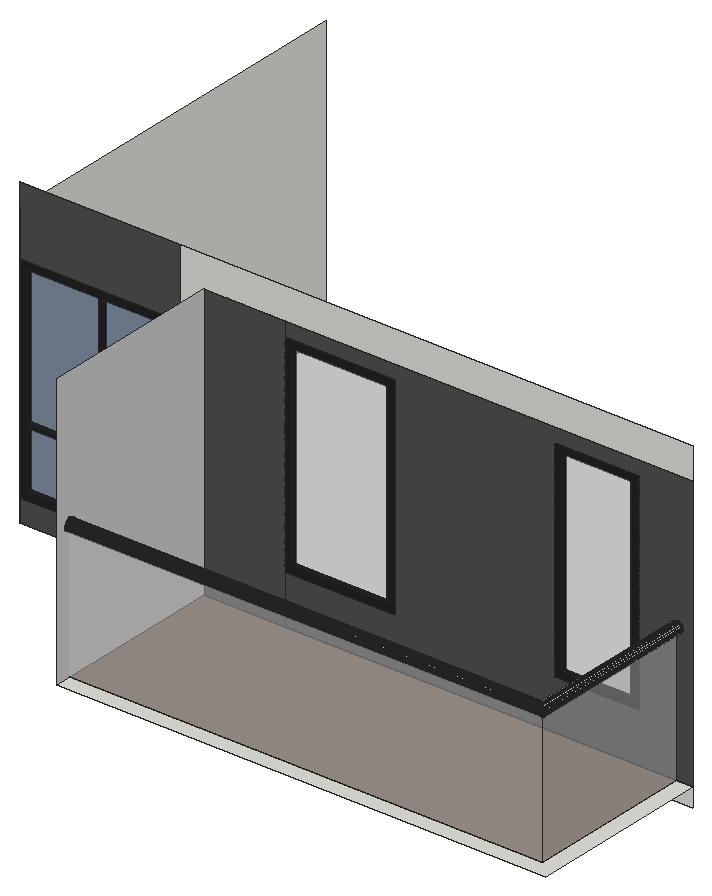
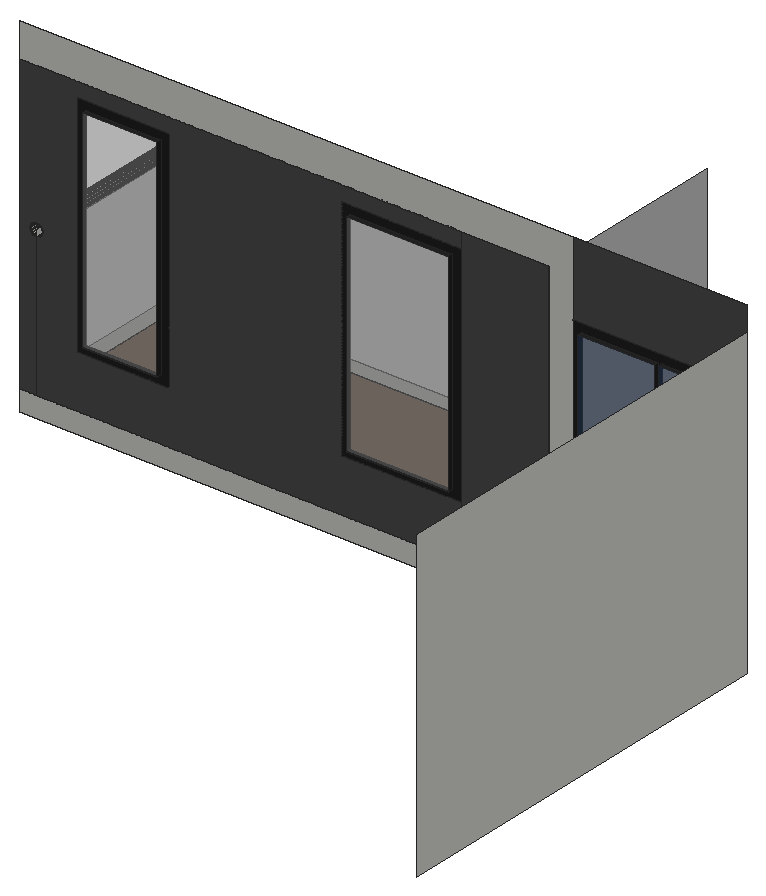
# SketchUp Ruby script. Lengths in inches.
U = 1.inch
M = Sketchup.active_model
def pt(a) = Geom::Point3d.new(a.map { |v| v * U })
def face(e, loops, mat)
  f = e.add_face(loops[0].map { |a| pt(a) })
  loops[1..].each { |l| e.add_face(l.map { |a| pt(a) }).erase! }
  f.material = f.back_material = mat if mat
  f
end
# faces: each face lists its corners as indices into pts; further lists are holes
def faces(e, pts, list, mat = nil) = list.each { |f| face(e, (f[0].is_a?(Array) ? f : [f]).map { |l| l.map { |i| pts[i] } }, mat) }
# xy, xz, yz: faces in a plane at the given z, y or x. An outline is a flat list of corners, or four numbers for a rectangle; further outlines are holes
def ring(l) = l.size == 4 ? [[l[0], l[1]], [l[2], l[1]], [l[2], l[3]], [l[0], l[3]]] : l.each_slice(2).to_a
def flat(e, list, mat, &to3) = list.each { |f| face(e, (f[0].is_a?(Array) ? f : [f]).map { |l| ring(l).map { |u, v| to3.(u, v) } }, mat) }
def xy(e, z, list, mat = nil) = flat(e, list, mat) { |x, y| [x, y, z] }
def xz(e, y, list, mat = nil) = flat(e, list, mat) { |x, z| [x, y, z] }
def yz(e, x, list, mat = nil) = flat(e, list, mat) { |y, z| [x, y, z] }
def lines(e, pts, list) = list.each { |a, b| e.add_line(pt(pts[a]), pt(pts[b])) }
# prism: a flat outline (further loops are holes) pulled along v
def prism(e, loops, v, mat = nil)
  f = face(e, loops, mat); d = Geom::Vector3d.new(v.map { |x| x * U })
  f.pushpull(f.normal.samedirection?(d) ? d.length : -d.length)
end
def box(e, o, s, mat = nil) = prism(e, [[o, [o[0] + s[0], o[1], o[2]], [o[0] + s[0], o[1] + s[1], o[2]], [o[0], o[1] + s[1], o[2]]]], [0, 0, s[2]], mat)
def at(x, y, z, deg = 0) = Geom::Transformation.translation(pt([x, y, z])) * Geom::Transformation.rotation(ORIGIN, Z_AXIS, deg.degrees)
def axes(o, x, y, z) = Geom::Transformation.new([*x, 0, *y, 0, *z, 0, *pt(o).to_a, 1])
def part(name) = M.definitions.add(name)
# library, detail: a bought-in or finely detailed component or shape, given as its bounding box
def library(name, o, s) = part(name).tap { |d| box(d.entities, o, s) }
def detail(e, o, s) = box(e.add_group.entities, o, s)
def put(e, d, t, mat = nil) = e.add_instance(d, t).tap { |i| i.material = mat if mat }
def group(e, t, mat = nil) = e.add_group.tap { |g| g.transformation = t; g.material = mat if mat }.entities
root = M.entities
M.materials.add("[0136_Charcoal]").color = [35, 35, 35]
M.materials.add("[Cladding Siding White]2").color = [81, 81, 81]
M.materials.add("[Cladding Siding White]3").color = [207, 207, 207]
M.materials.add("[Granite Brown]").color = [126, 104, 91]
M.materials.add("[Translucent Glass Blue]").color = [52, 78, 124]
M.materials["[Translucent Glass Blue]"].alpha = 0.5
M.materials.add("[Translucent Glass Gray]").color = [211, 211, 211]
M.materials["[Translucent Glass Gray]"].alpha = 0.5
M.materials.add("[Translucent Glass Gray]1").color = [163, 163, 163]
M.materials["[Translucent Glass Gray]1"].alpha = 0.5
xy(root,883.9375,[[559.63,120.38,558.375,120.39,557.125,120.53,555.9,120.8,554.71,121.2,553.5625,121.72,552.48,122.35,551.47,123.1,550.54,123.95,549.71,124.89,548.98,125.91,548.36,127,547.86,128.15,547.48,129.35,547.23,130.58,547.1,131.83,547.11,133.09,547.25,134.33,547.52,135.56,547.92,136.75,548.44,137.9,549.08,138.98,549.82,139.99,550.67,140.92,551.61,141.75,552.63,142.48,553.72,143.1,554.875,143.6,556.07,143.98,557.3,144.23,558.55,144.35,559.81,144.35,561.06,144.2,562.28,143.93,563.48,143.54,564.62,143.02,565.7,142.38,566.71,141.64,567.64,140.79,568.47,139.85,569.2,138.83,569.82,137.73,570.33,136.58,570.71,135.39,570.96,134.15,571.08,132.9,571.07,131.65,570.93,130.4,570.66,129.17,570.26,127.98,569.74,126.84,569.11,125.76,568.36,124.74,567.51,123.82,566.57,122.98,565.55,122.25,564.46,121.63,563.31,121.13,562.11,120.75,560.88,120.5],[937.5,120.38,936.25,120.39,935,120.53,933.77,120.8,932.58,121.2,931.4375,121.72,930.36,122.35,929.34,123.1,928.42,123.95,927.58,124.89,926.85,125.91,926.23,127,925.73,128.15,925.35,129.35,925.1,130.58,924.98,131.83,924.99,133.09,925.13,134.33,925.4,135.56,925.8,136.75,926.32,137.9,926.95,138.98,927.7,139.99,928.55,140.92,929.49,141.75,930.51,142.48,931.6,143.1,932.75,143.6,933.95,143.98,935.18,144.23,936.43,144.35,937.69,144.35,938.93,144.2,940.16,143.93,941.35,143.54,942.5,143.02,943.58,142.38,944.59,141.64,945.52,140.79,946.35,139.85,947.08,138.83,947.7,137.73,948.2,136.58,948.58,135.39,948.83,134.15,948.95,132.9,948.95,131.65,948.8,130.4,948.53,129.17,948.14,127.98,947.62,126.84,946.98,125.76,946.24,124.74,945.39,123.82,944.45,122.98,943.43,122.25,942.33,121.63,941.18,121.13,939.98,120.75,938.75,120.5]])
xy(root,936,[[348,0,1116,0,1116,288,1092.15,288,1092.15,24,348,24]])
xy(root,936,[[348,24,1092.15,288]],"[Granite Brown]")
xy(root,984,[[72,288,183,294],[189,288,300,294]],"[0136_Charcoal]")
xy(root,1025.88,[[487.9375,288,636,294],[912,288,1020,294]],"[0136_Charcoal]")
xy(root,1074,[[72,288,183,294],[189,288,300,294]],"[0136_Charcoal]")
xy(root,1080,[[72,288,183,294],[189,288,300,294]],"[0136_Charcoal]")
xy(root,1296,[[72,288,183,294],[189,288,300,294]],"[0136_Charcoal]")
xy(root,1332,[[487.9375,288,636,294],[912,288,1020,294]],"[0136_Charcoal]")
xz(root,24,[[348,1143,1092.15,1152]])
xz(root,24,[[348,936,1092.15,1143]],"[Translucent Glass Gray]")
xz(root,288,[[312,906,1116,936],[312,936,312,1416,1116,1416,1116,1366.34,348,1366.34,348,936]])
xz(root,288,[[[60,972,312,1308],[189,1080,300,1296],[72,1080,183,1296],[189,984,300,1074],[72,984,183,1074]],[[475.9375,1013.88,648,1344],[487.9375,1025.88,636,1332]],[[900,1013.88,1032,1344],[912,1025.88,1020,1332]]],"[0136_Charcoal]")
xz(root,288,[[60,936,312,972],[348,936,475.9375,1366.34],[[475.9375,936,1116,936,1116,1366.34,475.9375,1366.34,475.9375,1344,648,1344,648,1013.88,475.9375,1013.88],[900,1013.88,1032,1344],[1092.15,1143,1091.21,1143.05,1090.28,1143.2,1089.37,1143.44,1088.49,1143.78,1087.65,1144.21,1086.86,1144.72,1086.125,1145.3125,1085.46,1145.98,1084.87,1146.71,1084.35,1147.5,1083.92,1148.34,1083.59,1149.22,1083.34,1150.13,1083.2,1151.06,1083.15,1152,1083.2,1152.94,1083.34,1153.87,1083.59,1154.78,1083.92,1155.66,1084.35,1156.5,1084.87,1157.29,1085.46,1158.02,1086.125,1158.6875,1086.86,1159.28,1087.65,1159.79,1088.49,1160.22,1089.37,1160.56,1090.28,1160.8,1091.21,1160.95,1092.15,1161,1093.09,1160.95,1094.02,1160.8,1094.93,1160.56,1095.81,1160.22,1096.65,1159.79,1097.4375,1159.28,1098.17,1158.6875,1098.83,1158.02,1099.43,1157.29,1099.94,1156.5,1100.37,1155.66,1100.71,1154.78,1100.95,1153.87,1101.1,1152.94,1101.15,1152,1101.1,1151.06,1100.95,1150.13,1100.71,1149.22,1100.37,1148.34,1099.94,1147.5,1099.43,1146.71,1098.83,1145.98,1098.17,1145.3125,1097.4375,1144.72,1096.65,1144.21,1095.81,1143.78,1094.93,1143.44,1094.02,1143.2,1093.09,1143.05]],[60,1308,312,1416]],"[Cladding Siding White]2")
xz(root,294,[[72,984,183,1074],[189,984,300,1074],[72,1080,183,1296],[189,1080,300,1296]],"[Translucent Glass Blue]")
xz(root,294,[[487.9375,1025.88,636,1332],[912,1025.88,1020,1332]],"[Translucent Glass Gray]1")
yz(root,60,[[288,936,888,1380]])
yz(root,72,[[288,984,294,1074],[288,1080,294,1296]],"[0136_Charcoal]")
yz(root,183,[[288,984,294,1074],[288,1080,294,1296]],"[0136_Charcoal]")
yz(root,189,[[288,984,294,1074],[288,1080,294,1296]],"[0136_Charcoal]")
yz(root,300,[[288,984,294,1074],[288,1080,294,1296]],"[0136_Charcoal]")
yz(root,348,[[24,1143,23.06,1143.05,22.13,1143.2,21.22,1143.44,20.34,1143.78,19.5,1144.21,18.71,1144.72,17.98,1145.3125,17.3125,1145.98,16.72,1146.71,16.21,1147.5,15.78,1148.34,15.44,1149.22,15.2,1150.13,15.05,1151.06,15,1152,15.05,1152.94,15.2,1153.87,15.44,1154.78,15.78,1155.66,16.21,1156.5,16.72,1157.29,17.3125,1158.02,17.98,1158.6875,18.71,1159.28,19.5,1159.79,20.34,1160.22,21.22,1160.56,22.13,1160.8,23.06,1160.95,24,1161,24.94,1160.95,25.87,1160.8,26.78,1160.56,27.66,1160.22,28.5,1159.79,29.29,1159.28,30.02,1158.6875,30.6875,1158.02,31.28,1157.29,31.79,1156.5,32.22,1155.66,32.56,1154.78,32.8,1153.87,32.95,1152.94,33,1152,32.95,1151.06,32.8,1150.13,32.56,1149.22,32.22,1148.34,31.79,1147.5,31.28,1146.71,30.6875,1145.98,30.02,1145.3125,29.29,1144.72,28.5,1144.21,27.66,1143.78,26.78,1143.44,25.87,1143.2,24.94,1143.05]])
yz(root,348,[[[0,936,288,1366.34],[24,1143,23.06,1143.05,22.13,1143.2,21.22,1143.44,20.34,1143.78,19.5,1144.21,18.71,1144.72,17.98,1145.3125,17.3125,1145.98,16.72,1146.71,16.21,1147.5,15.78,1148.34,15.44,1149.22,15.2,1150.13,15.05,1151.06,15,1152,15.05,1152.94,15.2,1153.87,15.44,1154.78,15.78,1155.66,16.21,1156.5,16.72,1157.29,17.3125,1158.02,17.98,1158.6875,18.71,1159.28,19.5,1159.79,20.34,1160.22,21.22,1160.56,22.13,1160.8,23.06,1160.95,24,1161,24.94,1160.95,25.87,1160.8,26.78,1160.56,27.66,1160.22,28.5,1159.79,29.29,1159.28,30.02,1158.6875,30.6875,1158.02,31.28,1157.29,31.79,1156.5,32.22,1155.66,32.56,1154.78,32.8,1153.87,32.95,1152.94,33,1152,32.95,1151.06,32.8,1150.13,32.56,1149.22,32.22,1148.34,31.79,1147.5,31.28,1146.71,30.6875,1145.98,30.02,1145.3125,29.29,1144.72,28.5,1144.21,27.66,1143.78,26.78,1143.44,25.87,1143.2,24.94,1143.05]]],"[Cladding Siding White]3")
yz(root,487.9375,[[288,1025.88,294,1332]],"[0136_Charcoal]")
yz(root,636,[[288,1025.88,294,1332]],"[0136_Charcoal]")
yz(root,912,[[288,1025.88,294,1332]],"[0136_Charcoal]")
yz(root,1020,[[288,1025.88,294,1332]],"[0136_Charcoal]")
yz(root,1092.15,[[24,1143,288,1152]])
yz(root,1092.15,[[24,936,288,1143]],"[Translucent Glass Gray]")
p = [[348,22.13,1143.2],[348,23.06,1143.05],[1093.09,23.06,1143.05],[1094.02,22.13,1143.2],[1093.09,288,1143.05],[1094.02,288,1143.2],
  [348,24,1143],[1092.15,24,1143],[1092.15,288,1143],[348,24.94,1143.05],[1091.21,24.94,1143.05],[1091.21,288,1143.05],
  [348,25.87,1143.2],[1090.28,25.87,1143.2],[1090.28,288,1143.2],[348,21.22,1143.44],[1094.93,21.22,1143.44],[1094.93,288,1143.44],
  [348,26.78,1143.44],[1089.37,26.78,1143.44],[1089.37,288,1143.44],[348,20.34,1143.78],[1095.81,20.34,1143.78],[1095.81,288,1143.78],
  [348,27.66,1143.78],[1088.49,27.66,1143.78],[1088.49,288,1143.78],[348,19.5,1144.21],[1096.65,19.5,1144.21],[1096.65,288,1144.21],
  [348,28.5,1144.21],[1087.65,28.5,1144.21],[1087.65,288,1144.21],[348,18.71,1144.72],[1097.4375,18.71,1144.72],[1097.4375,288,1144.72],
  [348,29.29,1144.72],[1086.86,29.29,1144.72],[1086.86,288,1144.72],[348,17.98,1145.3125],[1098.17,17.98,1145.3125],[1098.17,288,1145.3125],
  [348,30.02,1145.3125],[1086.125,30.02,1145.3125],[1086.125,288,1145.3125],[348,17.3125,1145.98],[1098.83,17.3125,1145.98],[1098.83,288,1145.98],
  [348,30.6875,1145.98],[1085.46,30.6875,1145.98],[1085.46,288,1145.98],[348,16.72,1146.71],[1099.43,16.72,1146.71],[1099.43,288,1146.71],
  [348,31.28,1146.71],[1084.87,31.28,1146.71],[1084.87,288,1146.71],[348,16.21,1147.5],[1099.94,16.21,1147.5],[1099.94,288,1147.5],
  [348,31.79,1147.5],[1084.35,31.79,1147.5],[1084.35,288,1147.5],[348,15.78,1148.34],[1100.37,15.78,1148.34],[1100.37,288,1148.34],
  [348,32.22,1148.34],[1083.92,32.22,1148.34],[1083.92,288,1148.34],[348,15.44,1149.22],[1100.71,15.44,1149.22],[1100.71,288,1149.22],
  [348,32.56,1149.22],[1083.59,32.56,1149.22],[1083.59,288,1149.22],[348,15.2,1150.13],[1100.95,15.2,1150.13],[1100.95,288,1150.13],
  [348,32.8,1150.13],[1083.34,32.8,1150.13],[1083.34,288,1150.13],[348,15.05,1151.06],[1101.1,15.05,1151.06],[1101.1,288,1151.06],
  [348,32.95,1151.06],[1083.2,32.95,1151.06],[1083.2,288,1151.06],[348,15,1152],[1101.15,15,1152],[1101.15,288,1152],
  [348,33,1152],[1083.15,33,1152],[1083.15,288,1152],[348,15.05,1152.94],[1101.1,15.05,1152.94],[1101.1,288,1152.94],
  [348,32.95,1152.94],[1083.2,32.95,1152.94],[1083.2,288,1152.94],[348,15.2,1153.87],[1100.95,15.2,1153.87],[1100.95,288,1153.87],
  [348,32.8,1153.87],[1083.34,32.8,1153.87],[1083.34,288,1153.87],[348,15.44,1154.78],[1100.71,15.44,1154.78],[1100.71,288,1154.78],
  [348,32.56,1154.78],[1083.59,32.56,1154.78],[1083.59,288,1154.78],[348,15.78,1155.66],[1100.37,15.78,1155.66],[1100.37,288,1155.66],
  [348,32.22,1155.66],[1083.92,32.22,1155.66],[1083.92,288,1155.66],[348,16.21,1156.5],[1099.94,16.21,1156.5],[1099.94,288,1156.5],
  [348,31.79,1156.5],[1084.35,31.79,1156.5],[1084.35,288,1156.5],[348,16.72,1157.29],[1099.43,16.72,1157.29],[1099.43,288,1157.29],
  [348,31.28,1157.29],[1084.87,31.28,1157.29],[1084.87,288,1157.29],[348,17.3125,1158.02],[1098.83,17.3125,1158.02],[1098.83,288,1158.02],
  [348,30.6875,1158.02],[1085.46,30.6875,1158.02],[1085.46,288,1158.02],[348,17.98,1158.6875],[1098.17,17.98,1158.6875],[1098.17,288,1158.6875],
  [348,30.02,1158.6875],[1086.125,30.02,1158.6875],[1086.125,288,1158.6875],[348,18.71,1159.28],[1097.4375,18.71,1159.28],[1097.4375,288,1159.28],
  [348,29.29,1159.28],[1086.86,29.29,1159.28],[1086.86,288,1159.28],[348,19.5,1159.79],[1096.65,19.5,1159.79],[1096.65,288,1159.79],
  [348,28.5,1159.79],[1087.65,28.5,1159.79],[1087.65,288,1159.79],[348,20.34,1160.22],[1095.81,20.34,1160.22],[1095.81,288,1160.22],
  [348,27.66,1160.22],[1088.49,27.66,1160.22],[1088.49,288,1160.22],[348,21.22,1160.56],[1094.93,21.22,1160.56],[1094.93,288,1160.56],
  [348,26.78,1160.56],[1089.37,26.78,1160.56],[1089.37,288,1160.56],[348,22.13,1160.8],[1094.02,22.13,1160.8],[1094.02,288,1160.8],
  [348,25.87,1160.8],[1090.28,25.87,1160.8],[1090.28,288,1160.8],[348,23.06,1160.95],[1093.09,23.06,1160.95],[1093.09,288,1160.95],
  [348,24.94,1160.95],[1091.21,24.94,1160.95],[1091.21,288,1160.95],[348,24,1161],[1092.15,24,1161],[1092.15,288,1161]]
faces(root,p,[[0,1,2,3],[3,2,4,5],[1,6,7,2],[2,7,8,4],[6,9,10,7],[7,10,11,8],[9,12,13,10],[10,13,14,11],
  [15,0,3,16],[16,3,5,17],[12,18,19,13],[13,19,20,14],[21,15,16,22],[22,16,17,23],[18,24,25,19],[19,25,26,20],
  [27,21,22,28],[28,22,23,29],[24,30,31,25],[25,31,32,26],[33,27,28,34],[34,28,29,35],[30,36,37,31],[31,37,38,32],
  [39,33,34,40],[40,34,35,41],[36,42,43,37],[37,43,44,38],[45,39,40,46],[46,40,41,47],[42,48,49,43],[43,49,50,44],
  [51,45,46,52],[52,46,47,53],[48,54,55,49],[49,55,56,50],[57,51,52,58],[58,52,53,59],[54,60,61,55],[55,61,62,56],
  [63,57,58,64],[64,58,59,65],[60,66,67,61],[61,67,68,62],[69,63,64,70],[70,64,65,71],[66,72,73,67],[67,73,74,68],
  [75,69,70,76],[76,70,71,77],[72,78,79,73],[73,79,80,74],[81,75,76,82],[82,76,77,83],[78,84,85,79],[79,85,86,80],
  [87,81,82,88],[88,82,83,89],[84,90,91,85],[85,91,92,86],[93,87,88,94],[94,88,89,95],[90,96,97,91],[91,97,98,92],
  [99,93,94,100],[100,94,95,101],[96,102,103,97],[97,103,104,98],[105,99,100,106],[106,100,101,107],[102,108,109,103],[103,109,110,104],
  [111,105,106,112],[112,106,107,113],[108,114,115,109],[109,115,116,110],[117,111,112,118],[118,112,113,119],[114,120,121,115],[115,121,122,116],
  [123,117,118,124],[124,118,119,125],[120,126,127,121],[121,127,128,122],[129,123,124,130],[130,124,125,131],[126,132,133,127],[127,133,134,128],
  [135,129,130,136],[136,130,131,137],[132,138,139,133],[133,139,140,134],[141,135,136,142],[142,136,137,143],[138,144,145,139],[139,145,146,140],
  [147,141,142,148],[148,142,143,149],[144,150,151,145],[145,151,152,146],[153,147,148,154],[154,148,149,155],[150,156,157,151],[151,157,158,152],
  [159,153,154,160],[160,154,155,161],[156,162,163,157],[157,163,164,158],[165,159,160,166],[166,160,161,167],[162,168,169,163],[163,169,170,164],
  [171,165,166,172],[172,166,167,173],[168,174,175,169],[169,175,176,170],[177,171,172,178],[178,172,173,179],[174,177,178,175],[175,178,179,176]])
